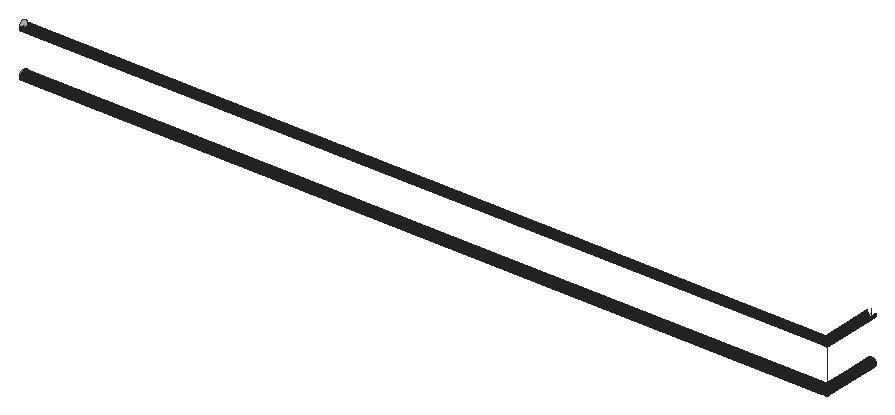
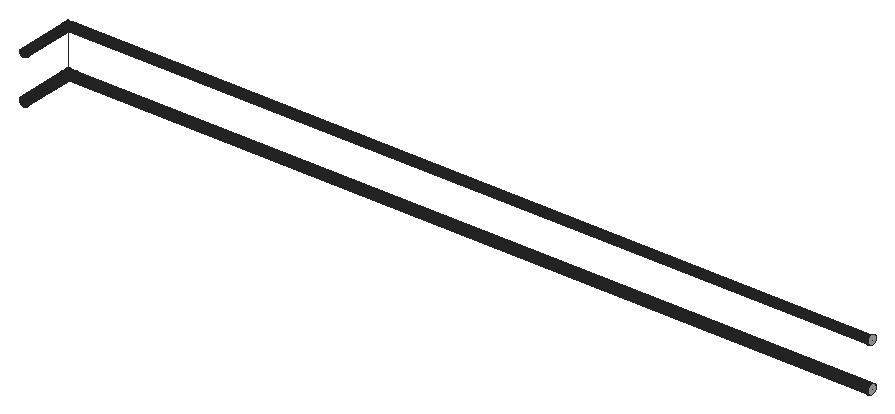
# SketchUp Ruby script. Lengths in inches.
U = 1.inch
M = Sketchup.active_model
def pt(a) = Geom::Point3d.new(a.map { |v| v * U })
def face(e, loops, mat)
  f = e.add_face(loops[0].map { |a| pt(a) })
  loops[1..].each { |l| e.add_face(l.map { |a| pt(a) }).erase! }
  f.material = f.back_material = mat if mat
  f
end
# faces: each face lists its corners as indices into pts; further lists are holes
def faces(e, pts, list, mat = nil) = list.each { |f| face(e, (f[0].is_a?(Array) ? f : [f]).map { |l| l.map { |i| pts[i] } }, mat) }
# xy, xz, yz: faces in a plane at the given z, y or x. An outline is a flat list of corners, or four numbers for a rectangle; further outlines are holes
def ring(l) = l.size == 4 ? [[l[0], l[1]], [l[2], l[1]], [l[2], l[3]], [l[0], l[3]]] : l.each_slice(2).to_a
def flat(e, list, mat, &to3) = list.each { |f| face(e, (f[0].is_a?(Array) ? f : [f]).map { |l| ring(l).map { |u, v| to3.(u, v) } }, mat) }
def xy(e, z, list, mat = nil) = flat(e, list, mat) { |x, y| [x, y, z] }
def xz(e, y, list, mat = nil) = flat(e, list, mat) { |x, z| [x, y, z] }
def yz(e, x, list, mat = nil) = flat(e, list, mat) { |y, z| [x, y, z] }
def lines(e, pts, list) = list.each { |a, b| e.add_line(pt(pts[a]), pt(pts[b])) }
# prism: a flat outline (further loops are holes) pulled along v
def prism(e, loops, v, mat = nil)
  f = face(e, loops, mat); d = Geom::Vector3d.new(v.map { |x| x * U })
  f.pushpull(f.normal.samedirection?(d) ? d.length : -d.length)
end
def box(e, o, s, mat = nil) = prism(e, [[o, [o[0] + s[0], o[1], o[2]], [o[0] + s[0], o[1] + s[1], o[2]], [o[0], o[1] + s[1], o[2]]]], [0, 0, s[2]], mat)
def at(x, y, z, deg = 0) = Geom::Transformation.translation(pt([x, y, z])) * Geom::Transformation.rotation(ORIGIN, Z_AXIS, deg.degrees)
def axes(o, x, y, z) = Geom::Transformation.new([*x, 0, *y, 0, *z, 0, *pt(o).to_a, 1])
def part(name) = M.definitions.add(name)
# library, detail: a bought-in or finely detailed component or shape, given as its bounding box
def library(name, o, s) = part(name).tap { |d| box(d.entities, o, s) }
def detail(e, o, s) = box(e.add_group.entities, o, s)
def put(e, d, t, mat = nil) = e.add_instance(d, t).tap { |i| i.material = mat if mat }
def group(e, t, mat = nil) = e.add_group.tap { |g| g.transformation = t; g.material = mat if mat }.entities
root = M.entities
M.materials.add("[0136_Charcoal]").color = [35, 35, 35]
yz(root,977.375,[[1090.62,2365,1089.78,2365.04,1088.95,2365.17,1088.15,2365.39,1087.36,2365.69,1086.62,2366.07,1085.92,2366.53,1085.26,2367.05,1084.67,2367.65,1084.15,2368.3,1083.6875,2369,1083.31,2369.75,1083.01,2370.53,1082.79,2371.34,1082.66,2372.16,1082.62,2373,1082.66,2373.84,1082.79,2374.66,1083.01,2375.47,1083.31,2376.25,1083.6875,2377,1084.15,2377.7,1084.67,2378.35,1085.26,2378.95,1085.92,2379.47,1086.62,2379.93,1087.36,2380.31,1088.15,2380.61,1088.95,2380.83,1089.78,2380.96,1090.62,2381,1091.45,2380.96,1092.28,2380.83,1093.09,2380.61,1093.87,2380.31,1094.62,2379.93,1095.32,2379.47,1095.97,2378.95,1096.5625,2378.35,1097.09,2377.7,1097.55,2377,1097.93,2376.25,1098.23,2375.47,1098.44,2374.66,1098.57,2373.84,1098.62,2373,1098.57,2372.16,1098.44,2371.34,1098.23,2370.53,1097.93,2369.75,1097.55,2369,1097.09,2368.3,1096.5625,2367.65,1095.97,2367.05,1095.32,2366.53,1094.62,2366.07,1093.87,2365.69,1093.09,2365.39,1092.28,2365.17,1091.45,2365.04],[1090.62,2446,1089.78,2446.04,1088.95,2446.17,1088.15,2446.39,1087.36,2446.69,1086.62,2447.07,1085.92,2447.53,1085.26,2448.05,1084.67,2448.65,1084.15,2449.3,1083.6875,2450,1083.31,2450.75,1083.01,2451.53,1082.79,2452.34,1082.66,2453.16,1082.62,2454,1082.66,2454.84,1082.79,2455.66,1083.01,2456.47,1083.31,2457.25,1083.6875,2458,1084.15,2458.7,1084.67,2459.35,1085.26,2459.95,1085.92,2460.47,1086.62,2460.93,1087.36,2461.31,1088.15,2461.61,1088.95,2461.83,1089.78,2461.96,1090.62,2462,1091.45,2461.96,1092.28,2461.83,1093.09,2461.61,1093.87,2461.31,1094.62,2460.93,1095.32,2460.47,1095.97,2459.95,1096.5625,2459.35,1097.09,2458.7,1097.55,2458,1097.93,2457.25,1098.23,2456.47,1098.44,2455.66,1098.57,2454.84,1098.62,2454,1098.57,2453.16,1098.44,2452.34,1098.23,2451.53,1097.93,2450.75,1097.55,2450,1097.09,2449.3,1096.5625,2448.65,1095.97,2448.05,1095.32,2447.53,1094.62,2447.07,1093.87,2446.69,1093.09,2446.39,1092.28,2446.17,1091.45,2446.04]])
p = [[977.375,1088.95,2365.17],[977.375,1089.78,2365.04],[2440.17,1089.78,2365.04],[2448.96,1089.78,2365.04],[2449.79,1088.95,2365.17],[2440.3,1088.95,2365.17],
  [2448.96,1098.57,2365.04],[2448.96,1192.62,2365.04],[2449.79,1192.62,2365.17],[2449.79,1098.44,2365.17],[977.375,1090.62,2365],[2440.125,1090.62,2365],
  [2448.125,1090.62,2365],[2448.125,1098.62,2365],[2448.125,1192.62,2365],[977.375,1091.45,2365.04],[2440.17,1091.45,2365.04],[2447.29,1091.45,2365.04],
  [2447.29,1098.57,2365.04],[2447.29,1192.62,2365.04],[977.375,1092.28,2365.17],[2440.3,1092.28,2365.17],[2446.46,1092.28,2365.17],[2446.46,1098.44,2365.17],
  [2446.46,1192.62,2365.17],[977.375,1088.15,2365.39],[2450.6,1088.15,2365.39],[2440.51,1088.15,2365.39],[2450.6,1192.62,2365.39],[2450.6,1098.23,2365.39],
  [977.375,1093.09,2365.39],[2440.51,1093.09,2365.39],[2445.65,1093.09,2365.39],[2445.65,1098.23,2365.39],[2445.65,1192.62,2365.39],[977.375,1087.36,2365.69],
  [2451.38,1087.36,2365.69],[2440.81,1087.36,2365.69],[2451.38,1192.62,2365.69],[2451.38,1097.93,2365.69],[977.375,1093.87,2365.69],[2440.81,1093.87,2365.69],
  [2444.87,1093.87,2365.69],[2444.87,1097.93,2365.69],[2444.87,1192.62,2365.69],[977.375,1086.62,2366.07],[2452.125,1086.62,2366.07],[2441.19,1086.62,2366.07],
  [2452.125,1192.62,2366.07],[2452.125,1097.55,2366.07],[977.375,1094.62,2366.07],[2441.19,1094.62,2366.07],[2444.125,1094.62,2366.07],[2444.125,1097.55,2366.07],
  [2444.125,1192.62,2366.07],[977.375,1085.92,2366.53],[2452.83,1085.92,2366.53],[2441.65,1085.92,2366.53],[2452.83,1192.62,2366.53],[2452.83,1097.09,2366.53],
  [977.375,1095.32,2366.53],[2441.65,1095.32,2366.53],[2443.42,1095.32,2366.53],[2443.42,1097.09,2366.53],[2443.42,1192.62,2366.53],[977.375,1085.26,2367.05],
  [2453.48,1085.26,2367.05],[2442.18,1085.26,2367.05],[2453.48,1192.62,2367.05],[2453.48,1096.5625,2367.05],[977.375,1095.97,2367.05],[2442.18,1095.97,2367.05],
  [2442.77,1095.97,2367.05],[2442.77,1096.5625,2367.05],[2442.77,1192.62,2367.05],[977.375,1084.67,2367.65],[2454.07,1084.67,2367.65],[2453.48,1084.67,2367.65],
  [2442.77,1084.67,2367.65],[2454.07,1192.62,2367.65],[2454.07,1095.97,2367.65],[2454.07,1085.26,2367.65],[977.375,1096.5625,2367.65],[2442.18,1096.5625,2367.65],
  [2442.18,1192.62,2367.65],[977.375,1084.15,2368.3],[2454.6,1084.15,2368.3],[2452.83,1084.15,2368.3],[2443.42,1084.15,2368.3],[2454.6,1192.62,2368.3],
  [2454.6,1095.32,2368.3],[2454.6,1085.92,2368.3],[977.375,1097.09,2368.3],[2441.65,1097.09,2368.3],[2441.65,1192.62,2368.3],[977.375,1083.6875,2369],
  [2455.05,1083.6875,2369],[2452.125,1083.6875,2369],[2444.125,1083.6875,2369],[2455.05,1192.62,2369],[2455.05,1094.62,2369],[2455.05,1086.62,2369],
  [977.375,1097.55,2369],[2441.19,1097.55,2369],[2441.19,1192.62,2369],[977.375,1083.31,2369.75],[2455.43,1083.31,2369.75],[2451.38,1083.31,2369.75],
  [2444.87,1083.31,2369.75],[2455.43,1192.62,2369.75],[2455.43,1093.87,2369.75],[2455.43,1087.36,2369.75],[977.375,1097.93,2369.75],[2440.81,1097.93,2369.75],
  [2440.81,1192.62,2369.75],[977.375,1083.01,2370.53],[2455.73,1083.01,2370.53],[2450.6,1083.01,2370.53],[2445.65,1083.01,2370.53],[2455.73,1192.62,2370.53],
  [2455.73,1093.09,2370.53],[2455.73,1088.15,2370.53],[977.375,1098.23,2370.53],[2440.51,1098.23,2370.53],[2440.51,1192.62,2370.53],[977.375,1082.79,2371.34],
  [2455.95,1082.79,2371.34],[2449.79,1082.79,2371.34],[2446.46,1082.79,2371.34],[2455.95,1192.62,2371.34],[2455.95,1092.28,2371.34],[2455.95,1088.95,2371.34],
  [977.375,1098.44,2371.34],[2440.3,1098.44,2371.34],[2440.3,1192.62,2371.34],[977.375,1082.66,2372.16],[2456.08,1082.66,2372.16],[2448.96,1082.66,2372.16],
  [2447.29,1082.66,2372.16],[2456.08,1192.62,2372.16],[2456.08,1091.45,2372.16],[2456.08,1089.78,2372.16],[977.375,1098.57,2372.16],[2440.17,1098.57,2372.16],
  [2440.17,1192.62,2372.16],[977.375,1082.62,2373],[2456.125,1082.62,2373],[2448.125,1082.62,2373],[2456.125,1192.62,2373],[2456.125,1090.62,2373],
  [977.375,1098.62,2373],[2440.125,1098.62,2373],[2440.125,1192.62,2373],[977.375,1082.66,2373.84],[2456.08,1082.66,2373.84],[2448.96,1082.66,2373.84],
  [2447.29,1082.66,2373.84],[2456.08,1192.62,2373.84],[2456.08,1091.45,2373.84],[2456.08,1089.78,2373.84],[977.375,1098.57,2373.84],[2440.17,1098.57,2373.84],
  [2440.17,1192.62,2373.84],[977.375,1082.79,2374.66],[2455.95,1082.79,2374.66],[2449.79,1082.79,2374.66],[2446.46,1082.79,2374.66],[2455.95,1192.62,2374.66],
  [2455.95,1092.28,2374.66],[2455.95,1088.95,2374.66],[977.375,1098.44,2374.66],[2440.3,1098.44,2374.66],[2440.3,1192.62,2374.66],[977.375,1083.01,2375.47],
  [2455.73,1083.01,2375.47],[2450.6,1083.01,2375.47],[2445.65,1083.01,2375.47],[2455.73,1192.62,2375.47],[2455.73,1093.09,2375.47],[2455.73,1088.15,2375.47],
  [977.375,1098.23,2375.47],[2440.51,1098.23,2375.47],[2440.51,1192.62,2375.47],[977.375,1083.31,2376.25],[2455.43,1083.31,2376.25],[2451.38,1083.31,2376.25],
  [2444.87,1083.31,2376.25],[2455.43,1192.62,2376.25],[2455.43,1093.87,2376.25],[2455.43,1087.36,2376.25],[977.375,1097.93,2376.25],[2440.81,1097.93,2376.25],
  [2440.81,1192.62,2376.25],[977.375,1083.6875,2377],[2455.05,1083.6875,2377],[2452.125,1083.6875,2377],[2444.125,1083.6875,2377],[2455.05,1192.62,2377],
  [2455.05,1094.62,2377],[2455.05,1086.62,2377],[977.375,1097.55,2377],[2441.19,1097.55,2377],[2441.19,1192.62,2377],[977.375,1084.15,2377.7],
  [2454.6,1084.15,2377.7],[2452.83,1084.15,2377.7],[2443.42,1084.15,2377.7],[2454.6,1192.62,2377.7],[2454.6,1095.32,2377.7],[2454.6,1085.92,2377.7],
  [977.375,1097.09,2377.7],[2441.65,1097.09,2377.7],[2441.65,1192.62,2377.7],[977.375,1084.67,2378.35],[2454.07,1084.67,2378.35],[2453.48,1084.67,2378.35],
  [2442.77,1084.67,2378.35],[2454.07,1192.62,2378.35],[2454.07,1095.97,2378.35],[2454.07,1085.26,2378.35],[977.375,1096.5625,2378.35],[2442.18,1096.5625,2378.35],
  [2442.18,1192.62,2378.35],[977.375,1085.26,2378.95],[2453.48,1085.26,2378.95],[2442.18,1085.26,2378.95],[2453.48,1192.62,2378.95],[2453.48,1096.5625,2378.95],
  [977.375,1095.97,2378.95],[2442.18,1095.97,2378.95],[2442.77,1095.97,2378.95],[2442.77,1096.5625,2378.95],[2442.77,1192.62,2378.95],[977.375,1085.92,2379.47],
  [2452.83,1085.92,2379.47],[2441.65,1085.92,2379.47],[2452.83,1192.62,2379.47],[2452.83,1097.09,2379.47],[977.375,1095.32,2379.47],[2441.65,1095.32,2379.47],
  [2443.42,1095.32,2379.47],[2443.42,1097.09,2379.47],[2443.42,1192.62,2379.47],[977.375,1086.62,2379.93],[2452.125,1086.62,2379.93],[2441.19,1086.62,2379.93],
  [2452.125,1192.62,2379.93],[2452.125,1097.55,2379.93],[977.375,1094.62,2379.93],[2441.19,1094.62,2379.93],[2444.125,1094.62,2379.93],[2444.125,1097.55,2379.93],
  [2444.125,1192.62,2379.93],[977.375,1087.36,2380.31],[2451.38,1087.36,2380.31],[2440.81,1087.36,2380.31],[2451.38,1192.62,2380.31],[2451.38,1097.93,2380.31],
  [977.375,1093.87,2380.31],[2440.81,1093.87,2380.31],[2444.87,1093.87,2380.31],[2444.87,1097.93,2380.31],[2444.87,1192.62,2380.31],[977.375,1088.15,2380.61],
  [2450.6,1088.15,2380.61],[2440.51,1088.15,2380.61],[2450.6,1192.62,2380.61],[2450.6,1098.23,2380.61],[977.375,1093.09,2380.61],[2440.51,1093.09,2380.61],
  [2445.65,1093.09,2380.61],[2445.65,1098.23,2380.61],[2445.65,1192.62,2380.61],[977.375,1088.95,2380.83],[2449.79,1088.95,2380.83],[2440.3,1088.95,2380.83],
  [2449.79,1192.62,2380.83],[2449.79,1098.44,2380.83],[977.375,1092.28,2380.83],[2440.3,1092.28,2380.83],[2446.46,1092.28,2380.83],[2446.46,1098.44,2380.83],
  [2446.46,1192.62,2380.83],[977.375,1089.78,2380.96],[2448.96,1089.78,2380.96],[2440.17,1089.78,2380.96],[2448.96,1192.62,2380.96],[2448.96,1098.57,2380.96],
  [977.375,1091.45,2380.96],[2440.17,1091.45,2380.96],[2447.29,1091.45,2380.96],[2447.29,1098.57,2380.96],[2447.29,1192.62,2380.96],[977.375,1090.62,2381],
  [2448.125,1090.62,2381],[2440.125,1090.62,2381],[2448.125,1192.62,2381],[2448.125,1098.62,2381],[977.375,1088.95,2446.17],[977.375,1089.78,2446.04],
  [2440.17,1089.78,2446.04],[2448.96,1089.78,2446.04],[2449.79,1088.95,2446.17],[2440.3,1088.95,2446.17],[2448.96,1098.57,2446.04],[2448.96,1192.62,2446.04],
  [2449.79,1192.62,2446.17],[2449.79,1098.44,2446.17],[977.375,1090.62,2446],[2440.125,1090.62,2446],[2448.125,1090.62,2446],[2448.125,1098.62,2446],
  [2448.125,1192.62,2446],[977.375,1091.45,2446.04],[2440.17,1091.45,2446.04],[2447.29,1091.45,2446.04],[2447.29,1098.57,2446.04],[2447.29,1192.62,2446.04],
  [977.375,1092.28,2446.17],[2440.3,1092.28,2446.17],[2446.46,1092.28,2446.17],[2446.46,1098.44,2446.17],[2446.46,1192.62,2446.17],[977.375,1088.15,2446.39],
  [2450.6,1088.15,2446.39],[2440.51,1088.15,2446.39],[2450.6,1192.62,2446.39],[2450.6,1098.23,2446.39],[977.375,1093.09,2446.39],[2440.51,1093.09,2446.39],
  [2445.65,1093.09,2446.39],[2445.65,1098.23,2446.39],[2445.65,1192.62,2446.39],[977.375,1087.36,2446.69],[2451.38,1087.36,2446.69],[2440.81,1087.36,2446.69],
  [2451.38,1192.62,2446.69],[2451.38,1097.93,2446.69],[977.375,1093.87,2446.69],[2440.81,1093.87,2446.69],[2444.87,1093.87,2446.69],[2444.87,1097.93,2446.69],
  [2444.87,1192.62,2446.69],[977.375,1086.62,2447.07],[2452.125,1086.62,2447.07],[2441.19,1086.62,2447.07],[2452.125,1192.62,2447.07],[2452.125,1097.55,2447.07],
  [977.375,1094.62,2447.07],[2441.19,1094.62,2447.07],[2444.125,1094.62,2447.07],[2444.125,1097.55,2447.07],[2444.125,1192.62,2447.07],[977.375,1085.92,2447.53],
  [2452.83,1085.92,2447.53],[2441.65,1085.92,2447.53],[2452.83,1192.62,2447.53],[2452.83,1097.09,2447.53],[977.375,1095.32,2447.53],[2441.65,1095.32,2447.53],
  [2443.42,1095.32,2447.53],[2443.42,1097.09,2447.53],[2443.42,1192.62,2447.53],[977.375,1085.26,2448.05],[2453.48,1085.26,2448.05],[2442.18,1085.26,2448.05],
  [2453.48,1192.62,2448.05],[2453.48,1096.5625,2448.05],[977.375,1095.97,2448.05],[2442.18,1095.97,2448.05],[2442.77,1095.97,2448.05],[2442.77,1096.5625,2448.05],
  [2442.77,1192.62,2448.05],[977.375,1084.67,2448.65],[2454.07,1084.67,2448.65],[2453.48,1084.67,2448.65],[2442.77,1084.67,2448.65],[2454.07,1192.62,2448.65],
  [2454.07,1095.97,2448.65],[2454.07,1085.26,2448.65],[977.375,1096.5625,2448.65],[2442.18,1096.5625,2448.65],[2442.18,1192.62,2448.65],[977.375,1084.15,2449.3],
  [2454.6,1084.15,2449.3],[2452.83,1084.15,2449.3],[2443.42,1084.15,2449.3],[2454.6,1192.62,2449.3],[2454.6,1095.32,2449.3],[2454.6,1085.92,2449.3],
  [977.375,1097.09,2449.3],[2441.65,1097.09,2449.3],[2441.65,1192.62,2449.3],[977.375,1083.6875,2450],[2455.05,1083.6875,2450],[2452.125,1083.6875,2450],
  [2444.125,1083.6875,2450],[2455.05,1192.62,2450],[2455.05,1094.62,2450],[2455.05,1086.62,2450],[977.375,1097.55,2450],[2441.19,1097.55,2450],
  [2441.19,1192.62,2450],[977.375,1083.31,2450.75],[2455.43,1083.31,2450.75],[2451.38,1083.31,2450.75],[2444.87,1083.31,2450.75],[2455.43,1192.62,2450.75],
  [2455.43,1093.87,2450.75],[2455.43,1087.36,2450.75],[977.375,1097.93,2450.75],[2440.81,1097.93,2450.75],[2440.81,1192.62,2450.75],[977.375,1083.01,2451.53],
  [2455.73,1083.01,2451.53],[2450.6,1083.01,2451.53],[2445.65,1083.01,2451.53],[2455.73,1192.62,2451.53],[2455.73,1093.09,2451.53],[2455.73,1088.15,2451.53],
  [977.375,1098.23,2451.53],[2440.51,1098.23,2451.53],[2440.51,1192.62,2451.53],[977.375,1082.79,2452.34],[2455.95,1082.79,2452.34],[2449.79,1082.79,2452.34],
  [2446.46,1082.79,2452.34],[2455.95,1192.62,2452.34],[2455.95,1092.28,2452.34],[2455.95,1088.95,2452.34],[977.375,1098.44,2452.34],[2440.3,1098.44,2452.34],
  [2440.3,1192.62,2452.34],[977.375,1082.66,2453.16],[2456.08,1082.66,2453.16],[2448.96,1082.66,2453.16],[2447.29,1082.66,2453.16],[2456.08,1192.62,2453.16],
  [2456.08,1091.45,2453.16],[2456.08,1089.78,2453.16],[977.375,1098.57,2453.16],[2440.17,1098.57,2453.16],[2440.17,1192.62,2453.16],[977.375,1082.62,2454],
  [2456.125,1082.62,2454],[2448.125,1082.62,2454],[2456.125,1192.62,2454],[2456.125,1090.62,2454],[977.375,1098.62,2454],[2440.125,1098.62,2454],
  [2440.125,1192.62,2454],[977.375,1082.66,2454.84],[2456.08,1082.66,2454.84],[2448.96,1082.66,2454.84],[2447.29,1082.66,2454.84],[2456.08,1192.62,2454.84],
  [2456.08,1091.45,2454.84],[2456.08,1089.78,2454.84],[977.375,1098.57,2454.84],[2440.17,1098.57,2454.84],[2440.17,1192.62,2454.84],[977.375,1082.79,2455.66],
  [2455.95,1082.79,2455.66],[2449.79,1082.79,2455.66],[2446.46,1082.79,2455.66],[2455.95,1192.62,2455.66],[2455.95,1092.28,2455.66],[2455.95,1088.95,2455.66],
  [977.375,1098.44,2455.66],[2440.3,1098.44,2455.66],[2440.3,1192.62,2455.66],[2448.125,1090.62,2454],[2448.125,1090.62,2462],[2440.125,1090.62,2454],
  [2448.125,1090.62,2373],[2440.125,1090.62,2373],[2448.125,1192.62,2454],[2448.125,1098.62,2454],[2448.125,1192.62,2373],[2448.125,1098.62,2373],
  [2448.125,1192.62,2462],[977.375,1090.62,2454],[977.375,1090.62,2373]]
faces(root,p,[[0,1,2,3,4,5],[4,3,6,7,8,9],[1,10,11,12,3,2],[3,12,13,14,7,6],[10,15,16,17,12,11],[12,17,18,19,14,13],[15,20,21,22,17,16],[17,22,23,24,19,18],
  [25,0,5,4,26,27],[26,4,9,8,28,29],[20,30,31,32,22,21],[22,32,33,34,24,23],[35,25,27,26,36,37],[36,26,29,28,38,39],[30,40,41,42,32,31],[32,42,43,44,34,33],
  [45,35,37,36,46,47],[46,36,39,38,48,49],[40,50,51,52,42,41],[42,52,53,54,44,43],[55,45,47,46,56,57],[56,46,49,48,58,59],[50,60,61,62,52,51],[52,62,63,64,54,53],
  [65,55,57,56,66,67],[66,56,59,58,68,69],[60,70,71,72,62,61],[62,72,73,74,64,63],[75,65,67,66,76,77,78],[76,66,69,68,79,80,81],[70,82,83,72,71],[72,83,84,74,73],
  [85,75,78,77,76,86,87,88],[86,76,81,80,79,89,90,91],[82,92,93,83],[83,93,94,84],[95,85,88,87,86,96,97,98],[96,86,91,90,89,99,100,101],[92,102,103,93],[93,103,104,94],
  [105,95,98,97,96,106,107,108],[106,96,101,100,99,109,110,111],[102,112,113,103],[103,113,114,104],[115,105,108,107,106,116,117,118],[116,106,111,110,109,119,120,121],[112,122,123,113],[113,123,124,114],
  [125,115,118,117,116,126,127,128],[126,116,121,120,119,129,130,131],[122,132,133,123],[123,133,134,124],[135,125,128,127,126,136,137,138],[136,126,131,130,129,139,140,141],[132,142,143,133],[133,143,144,134],
  [145,135,138,137,136,146,147],[146,136,141,140,139,148,149],[142,150,151,143],[143,151,152,144],[153,145,147,146,154,155,156],[154,146,149,148,157,158,159],[150,160,161,151],[151,161,162,152],
  [163,153,156,155,154,164,165,166],[164,154,159,158,157,167,168,169],[160,170,171,161],[161,171,172,162],[173,163,166,165,164,174,175,176],[174,164,169,168,167,177,178,179],[170,180,181,171],[171,181,182,172],
  [183,173,176,175,174,184,185,186],[184,174,179,178,177,187,188,189],[180,190,191,181],[181,191,192,182],[193,183,186,185,184,194,195,196],[194,184,189,188,187,197,198,199],[190,200,201,191],[191,201,202,192],
  [203,193,196,195,194,204,205,206],[204,194,199,198,197,207,208,209],[200,210,211,201],[201,211,212,202],[213,203,206,205,204,214,215,216],[214,204,209,208,207,217,218,219],[210,220,221,211],[211,221,222,212],
  [223,213,216,215,214,224,225],[224,214,219,218,217,226,227],[220,228,229,230,221],[221,230,231,232,222],[233,223,225,224,234,235],[234,224,227,226,236,237],[228,238,239,240,230,229],[230,240,241,242,232,231],
  [243,233,235,234,244,245],[244,234,237,236,246,247],[238,248,249,250,240,239],[240,250,251,252,242,241],[253,243,245,244,254,255],[254,244,247,246,256,257],[248,258,259,260,250,249],[250,260,261,262,252,251],
  [263,253,255,254,264,265],[264,254,257,256,266,267],[258,268,269,270,260,259],[260,270,271,272,262,261],[273,263,265,264,274,275],[274,264,267,266,276,277],[268,278,279,280,270,269],[270,280,281,282,272,271],
  [283,273,275,274,284,285],[284,274,277,276,286,287],[278,288,289,290,280,279],[280,290,291,292,282,281],[293,283,285,284,294,295],[294,284,287,286,296,297],[288,293,295,294,290,289],[290,294,297,296,292,291],
  [298,299,300,301,302,303],[302,301,304,305,306,307],[299,308,309,310,301,300],[301,310,311,312,305,304],[308,313,314,315,310,309],[310,315,316,317,312,311],[313,318,319,320,315,314],[315,320,321,322,317,316],
  [323,298,303,302,324,325],[324,302,307,306,326,327],[318,328,329,330,320,319],[320,330,331,332,322,321],[333,323,325,324,334,335],[334,324,327,326,336,337],[328,338,339,340,330,329],[330,340,341,342,332,331],
  [343,333,335,334,344,345],[344,334,337,336,346,347],[338,348,349,350,340,339],[340,350,351,352,342,341],[353,343,345,344,354,355],[354,344,347,346,356,357],[348,358,359,360,350,349],[350,360,361,362,352,351],
  [363,353,355,354,364,365],[364,354,357,356,366,367],[358,368,369,370,360,359],[360,370,371,372,362,361],[373,363,365,364,374,375,376],[374,364,367,366,377,378,379],[368,380,381,370,369],[370,381,382,372,371],
  [383,373,376,375,374,384,385,386],[384,374,379,378,377,387,388,389],[380,390,391,381],[381,391,392,382],[393,383,386,385,384,394,395,396],[394,384,389,388,387,397,398,399],[390,400,401,391],[391,401,402,392],
  [403,393,396,395,394,404,405,406],[404,394,399,398,397,407,408,409],[400,410,411,401],[401,411,412,402],[413,403,406,405,404,414,415,416],[414,404,409,408,407,417,418,419],[410,420,421,411],[411,421,422,412],
  [423,413,416,415,414,424,425,426],[424,414,419,418,417,427,428,429],[420,430,431,421],[421,431,432,422],[433,423,426,425,424,434,435,436],[434,424,429,428,427,437,438,439],[430,440,441,431],[431,441,442,432],
  [443,433,436,435,434,444,445],[444,434,439,438,437,446,447],[440,448,449,441],[441,449,450,442],[451,443,445,444,452,453,454],[452,444,447,446,455,456,457],[448,458,459,449],[449,459,460,450],
  [461,451,454,453,452,462,463,464],[462,452,457,456,455,465,466,467],[458,468,469,459],[459,469,470,460]],"[0136_Charcoal]")
lines(root,p,[[471,472],[471,473],[474,294],[474,475],[476,312],[471,477],[478,14],[474,479],[310,471],[480,476],[12,474],[294,310],
  [296,478],[473,481],[475,482],[477,476],[479,478]])
